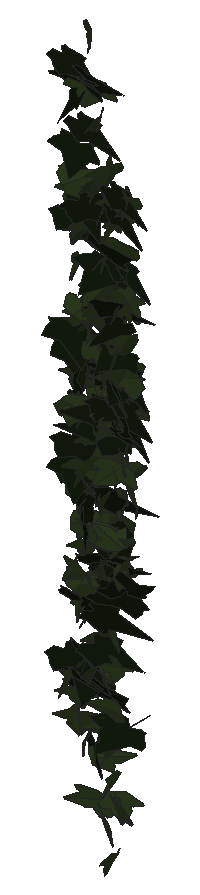
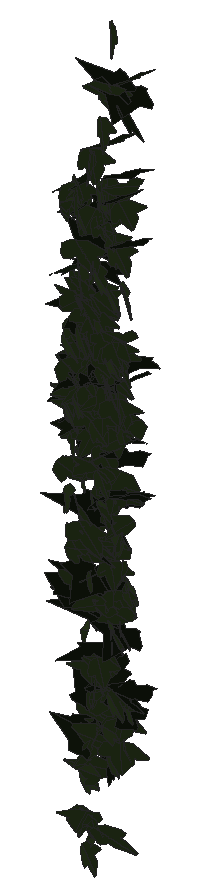
# SketchUp Ruby script. Lengths in millimetres.
U = 1.mm
M = Sketchup.active_model
def pt(a) = Geom::Point3d.new(a.map { |v| v * U })
def face(e, loops, mat)
  f = e.add_face(loops[0].map { |a| pt(a) })
  loops[1..].each { |l| e.add_face(l.map { |a| pt(a) }).erase! }
  f.material = f.back_material = mat if mat
  f
end
# faces: each face lists its corners as indices into pts; further lists are holes
def faces(e, pts, list, mat = nil) = list.each { |f| face(e, (f[0].is_a?(Array) ? f : [f]).map { |l| l.map { |i| pts[i] } }, mat) }
# xy, xz, yz: faces in a plane at the given z, y or x. An outline is a flat list of corners, or four numbers for a rectangle; further outlines are holes
def ring(l) = l.size == 4 ? [[l[0], l[1]], [l[2], l[1]], [l[2], l[3]], [l[0], l[3]]] : l.each_slice(2).to_a
def flat(e, list, mat, &to3) = list.each { |f| face(e, (f[0].is_a?(Array) ? f : [f]).map { |l| ring(l).map { |u, v| to3.(u, v) } }, mat) }
def xy(e, z, list, mat = nil) = flat(e, list, mat) { |x, y| [x, y, z] }
def xz(e, y, list, mat = nil) = flat(e, list, mat) { |x, z| [x, y, z] }
def yz(e, x, list, mat = nil) = flat(e, list, mat) { |y, z| [x, y, z] }
def lines(e, pts, list) = list.each { |a, b| e.add_line(pt(pts[a]), pt(pts[b])) }
# prism: a flat outline (further loops are holes) pulled along v
def prism(e, loops, v, mat = nil)
  f = face(e, loops, mat); d = Geom::Vector3d.new(v.map { |x| x * U })
  f.pushpull(f.normal.samedirection?(d) ? d.length : -d.length)
end
def box(e, o, s, mat = nil) = prism(e, [[o, [o[0] + s[0], o[1], o[2]], [o[0] + s[0], o[1] + s[1], o[2]], [o[0], o[1] + s[1], o[2]]]], [0, 0, s[2]], mat)
def at(x, y, z, deg = 0) = Geom::Transformation.translation(pt([x, y, z])) * Geom::Transformation.rotation(ORIGIN, Z_AXIS, deg.degrees)
def axes(o, x, y, z) = Geom::Transformation.new([*x, 0, *y, 0, *z, 0, *pt(o).to_a, 1])
def part(name) = M.definitions.add(name)
# library, detail: a bought-in or finely detailed component or shape, given as its bounding box
def library(name, o, s) = part(name).tap { |d| box(d.entities, o, s) }
def detail(e, o, s) = box(e.add_group.entities, o, s)
def put(e, d, t, mat = nil) = e.add_instance(d, t).tap { |i| i.material = mat if mat }
def group(e, t, mat = nil) = e.add_group.tap { |g| g.transformation = t; g.material = mat if mat }.entities
root = M.entities
M.materials.add("efeu1").color = [18, 25, 13]
M.materials.add("efeu2").color = [43, 57, 29]
c1 = part("ivyleaf_10")
p = [[0,12.8,-0.8],[-1.5,51.3,-10.9],[-4.9,51,-11.6],[-13.6,26.5,-7.3],[-13.2,15.9,-4.6],[-21.1,19.3,-7.2],
  [-29.5,16.3,-8.3],[-29.2,8.3,-6.2],[-19.7,-9.8,0.5],[-7.6,-13,4],[1,-12.2,5.8],[-0.4,51.1,-11.1],
  [-1.5,51.1,-10.9],[1,-12.4,5.9],[16.9,-12.4,3.5],[35.1,9.1,-5.1],[35,12.9,-6.1],[20.5,16.4,-4.9],
  [15.8,15,-3.8],[15.3,27.6,-7.1],[12.8,31.3,-7.8]]
faces(c1.entities,p,[[0,1,2,3,4,5,6,7,8,9,10],[11,12,0,13,14,15,16,17,18,19,20]],"efeu2")
c2 = part("ivyleaf_9")
p = [[39.1,54.8,31.7],[34.5,51.8,30.2],[-5.3,25.2,17.3],[-17.9,28.3,20.9],[-21.6,21.7,17],[-20.2,4.3,5.3],
  [-22.9,-0.3,2.5],[-17.1,-4,-0.6],[-2,-2.1,-1.2],[-0.7,-15.4,-10.1],[16.6,-22.3,-16.7],[21.1,-15.1,-12.5],
  [32.7,-10.7,-11],[46.1,-1.8,-6.6],[30.8,11.2,3.8]]
faces(c2.entities,p,[[0,1,2,3,4,5,6,7,8,9,10,11,12,13,14]],"efeu1")
put(root,c1,axes([1571.3,1015.9,668.1],[-0.2467,0.55616,-0.33098],[0.13791,-0.32296,-0.57106],[-1.22399,-0.14848,0.00237]))
put(root,c1,axes([1572.5,998.6,417.9],[0.27227,-0.40908,0.65552],[0.39143,-0.62245,-0.43333],[1.41754,0.25045,-0.00625]))
put(root,c1,axes([1567.8,1029,916.7],[-0.03546,-0.06959,0.70337],[0.65785,-0.61463,-0.05166],[1.17335,0.3425,0.05022]))
put(root,c1,axes([1580.5,1004,1147.2],[0.51099,-0.69659,-0.1656],[-0.05034,0.16709,-0.74574],[1.36176,0.26756,0.03457]))
put(root,c1,axes([1571.4,1008.6,747.9],[0.22223,0.32998,0.59583],[0.08777,0.5993,-0.34094],[-1.29329,0.09737,0.07924]))
put(root,c1,axes([1582.2,1024.8,1055.8],[-0.59959,-0.63157,0.16688],[0.03186,-0.19302,-0.69889],[1.24285,-0.29974,0.09842]))
put(root,c2,axes([1565.9,996.7,459.9],[0.02456,-0.40531,-0.66696],[0.0762,0.66651,-0.40426],[1.4834,-0.02753,0.03181]))
put(root,c1,axes([1588.2,1017.2,949.7],[-0.91985,-0.48124,0.19716],[-0.21237,-0.16693,-0.68099],[0.96674,-0.49457,0.03801]))
put(root,c1,axes([1590.5,1009.6,1027.6],[0.60365,-0.465,-0.45066],[-0.47859,0.37398,-0.56287],[1.1357,0.40476,0.00234]))
put(root,c1,axes([1596.5,991.9,612.7],[-0.91654,0.17381,0.41087],[-0.78506,0.05681,-0.50751],[-0.32341,-0.63048,0.06754]))
put(root,c2,axes([1565.1,1013.1,892.5],[0.76321,-0.45053,-0.46464],[-0.19004,0.49699,-0.56808],[1.21701,0.36015,0.20268]))
put(root,c1,axes([1583.8,1010.3,963.2],[0.10547,-0.61187,-0.33958],[0.00087,0.34067,-0.61377],[1.33183,0.04824,0.02729]))
put(root,c1,axes([1587.9,1017.7,1044.3],[-0.83524,-0.57309,0.04169],[-0.04203,-0.0356,-0.72181],[1.09278,-0.4394,0.00411]))
put(root,c1,axes([1587.8,1005.5,349],[-1.17604,-0.44909,0.02119],[-0.02351,-0.01904,-0.76384],[0.85533,-0.618,0.00814]))
put(root,c1,axes([1575.5,989.2,606.3],[0.26339,-0.66648,-0.11301],[0.11433,-0.10277,0.67967],[-1.28146,-0.14616,0.03741]))
put(root,c1,axes([1587,999.9,1288.4],[-0.53752,-0.66214,0.27353],[0.05023,-0.30344,-0.70728],[1.36255,-0.25002,0.13398]))
put(root,c1,axes([1589.3,1009.9,1217.6],[-0.27287,-0.74091,0.11093],[-0.08269,-0.10453,-0.75431],[1.42341,-0.14811,-0.02255]))
put(root,c2,axes([1568.6,1000.1,1235.9],[0.23567,-0.64879,-0.39765],[0.10163,0.4093,-0.65116],[1.44469,0.07704,0.11068]))
put(root,c2,axes([1576.8,1001.7,1031.5],[-0.70551,-0.6188,-0.35039],[0.3314,0.30413,-0.72131],[1.31219,-0.40951,-0.00623]))
put(root,c2,axes([1581.7,1007.6,1354.6],[-0.62223,-0.68562,0.137],[-0.02858,-0.14432,-0.75808],[1.33037,-0.32377,0.04779]))
put(root,c1,axes([1586.6,1000.9,394.3],[-1.05283,-0.3505,-0.07329],[0.1308,0.02845,-0.65476],[0.66884,-0.5573,0.01268]))
put(root,c1,axes([1587.9,1023.6,442.5],[0.18433,-0.70342,0.15714],[0.01915,-0.15722,-0.70997],[1.37161,0.09673,-0.01121]))
put(root,c2,axes([1574.7,1001.1,995.3],[-0.08397,-0.79522,-0.04255],[0.01864,0.04207,-0.79641],[1.51552,-0.04458,0.00744]))
put(root,c1,axes([1583.5,1021.2,717.2],[-0.12826,-0.12145,-0.66567],[-0.04806,-0.66804,0.12444],[-1.28692,0.03705,0.06169]))
put(root,c2,axes([1582.3,1002.9,789.2],[-0.56018,-0.71563,-0.02349],[0.00585,0.02413,-0.77377],[1.36271,-0.29428,-0.00633]))
put(root,c1,axes([1586.4,1023.7,560.4],[0.78746,-0.60576,0.09546],[0.07673,-0.08804,-0.7334],[1.16459,0.4154,-0.01623]))
put(root,c2,axes([1593.9,994.6,1457],[-0.93924,0.41452,-0.46805],[0.70275,-0.28796,-0.64435],[-0.96024,-0.6162,-0.01375]))
put(root,c2,axes([1581.6,1003.3,557.9],[1.39909,0.05142,-0.30835],[-0.586,-0.0172,-0.73691],[-0.10292,0.79699,0.00399]))
put(root,c1,axes([1608,1020.9,201.7],[0.70546,-0.02856,-0.60696],[-1.14695,0.07369,-0.3715],[0.14797,0.70737,0.0142]))
put(root,c1,axes([1591.6,1026,1038.5],[0.17746,-0.70303,0.1308],[-0.00469,-0.13222,-0.70892],[1.36096,0.09122,-0.0195]))
put(root,c2,axes([1569.1,986.4,1518.5],[0.61992,-0.67329,-0.30174],[0.10223,0.3506,-0.72433],[1.40047,0.27244,0.18644]))
put(root,c1,axes([1614.5,1006,995.7],[-0.65115,0.0281,0.67312],[-1.27638,0.05762,-0.34329],[-0.122,-0.75288,-0.00115]))
put(root,c1,axes([1573.3,1008.9,352.7],[0.49889,-0.2531,0.68432],[0.89549,-0.4971,-0.36409],[1.0613,0.53842,-0.01447]))
put(root,c1,axes([1580.2,1009.3,555.1],[0.65025,-0.49758,0.39293],[0.52117,-0.28676,-0.60125],[1.08831,0.43462,0.05315]))
put(root,c1,axes([1588.3,1003.6,706.9],[-0.61576,0.56651,-0.06615],[0.05381,-0.06003,-0.65237],[-1.08418,-0.32473,0.00519]))
put(root,c1,axes([1580.6,1005.9,1062.6],[0.63518,0.32461,-0.59421],[0.64135,0.49497,0.45966],[1.11772,-0.46848,0.07392]))
put(root,c2,axes([1592.5,980.9,1489.2],[1.27558,0.40751,-0.24645],[-0.58004,0.04008,-0.76257],[-0.69647,0.71298,0.18372]))
put(root,c1,axes([1595.2,1003.9,799.4],[-0.8837,-0.61169,-0.19589],[0.22243,0.15722,-0.76796],[1.202,-0.4788,-0.00191]))
put(root,c2,axes([1576.2,1003.4,793.3],[0.05356,-0.46715,-0.61659],[0.38556,0.59991,-0.44527],[1.42088,-0.14518,0.14407]))
put(root,c1,axes([1617.8,1006.7,790.2],[0.31984,0.13555,-0.7043],[-1.33673,-0.11542,-0.1898],[-0.27648,0.71482,0.10291]))
put(root,c1,axes([1597.6,1020,384.8],[0.0955,-0.44885,0.47814],[0.05266,-0.47767,-0.4513],[1.24703,0.05454,-0.01756]))
put(root,c2,axes([1565.9,1002.4,409.2],[0.66335,-0.25759,0.64088],[0.94752,-0.40389,-0.43309],[0.91119,0.60752,-0.0162]))
put(root,c1,axes([1601.8,999.5,767.3],[-0.70343,0.47797,0.25833],[-0.3528,0.18275,-0.60335],[-0.97199,-0.41224,0.03205]))
put(root,c1,axes([1602.2,1002.3,1224.4],[-0.12873,-0.69563,0.2869],[-0.05495,-0.28544,-0.69891],[1.43105,-0.07353,-0.00103]))
put(root,c1,axes([1594.3,1002.6,820.7],[-1.11835,-0.30404,-0.24429],[0.4034,0.12187,-0.66153],[0.62311,-0.62459,-0.01016]))
put(root,c1,axes([1601.8,992.3,1221.6],[-0.04665,-0.64527,-0.38576],[0.03603,0.38531,-0.64572],[1.43034,-0.03075,0.00369]))
put(root,c1,axes([1593.6,1020.9,1060.4],[-1.30245,0.04444,-0.22898],[0.42736,-0.06655,-0.68402],[-0.12013,-0.71856,0.04919]))
put(root,c1,axes([1603.3,1006.2,659.3],[-0.68482,-0.54915,-0.00647],[0.00771,0.00508,-0.65654],[1.0452,-0.35985,0.0006]))
put(root,c1,axes([1619.9,1013.9,423.1],[-0.0077,0.02322,0.68184],[-0.9832,-0.44547,0.01211],[0.84809,-0.51622,0.02022]))
put(root,c2,axes([1584.8,1000.5,1311.1],[0.2239,-0.7227,-0.23839],[0.07044,0.24637,-0.72862],[1.44662,0.09986,0.07237]))
put(root,c1,axes([1582.7,982,909.9],[-0.65632,-0.23576,-0.59298],[1.07831,0.19698,-0.40782],[0.55875,-0.65707,0.0905]))
put(root,c2,axes([1622.8,985.3,740.5],[-0.2949,0.04401,-0.79776],[-1.42065,0.28179,0.16053],[0.54221,0.76225,-0.01329]))
put(root,c1,axes([1605,989.6,900.5],[0.24019,-0.5809,-0.46086],[-0.02731,0.46549,-0.59066],[1.41098,0.1079,0.06702]))
put(root,c2,axes([1602.7,982.1,945.8],[-0.09331,-0.34116,0.7374],[0.63201,0.66581,0.33012],[-1.41128,0.32072,0.09908]))
put(root,c1,axes([1593.2,1009.1,887.5],[-0.86768,0.42668,-0.33487],[0.49644,-0.21107,-0.62406],[-0.90507,-0.52482,-0.02127]))
put(root,c1,axes([1606,997.7,796.2],[0.14635,-0.63436,0.29675],[0.02975,-0.29691,-0.63874],[1.33256,0.0763,-0.01833]))
put(root,c1,axes([1603.1,1011.6,975.8],[0.46632,-0.65295,0.10297],[0.12903,-0.08441,-0.69661],[1.25142,0.25202,0.03346]))
put(root,c1,axes([1585.2,1004.6,577.6],[0.85818,0.17818,-0.53629],[0.92631,0.22619,0.48438],[0.54654,-0.66315,0.02112]))
put(root,c1,axes([1591.3,969.3,1310.3],[0.40457,0.04788,-0.83473],[0.79836,0.73893,0.14921],[1.3765,-0.44265,0.15879]))
put(root,c1,axes([1598.2,1004,307],[0.13502,-0.52051,-0.47781],[0.118,-0.47378,0.52532],[-1.33955,-0.0942,-0.00189]))
put(root,c1,axes([1605.3,1014.2,939.5],[-1.23924,-0.28772,0.04328],[0.0754,0.01742,0.71187],[-0.54858,0.65234,0.00007]))
put(root,c2,axes([1591.3,983.4,851.5],[0.01509,-0.53012,-0.6409],[0.11299,0.63966,-0.52835],[1.57892,-0.04071,0.04393]))
put(root,c1,axes([1609.6,995.4,542],[0.06522,-0.53437,-0.42188],[-0.04824,0.42112,-0.53546],[1.29486,0.0426,0.0013]))
put(root,c1,axes([1609.7,1023.8,825.1],[-0.13731,-0.67541,0.00443],[-0.00083,-0.00441,-0.67925],[1.28547,-0.07215,0.00003]))
put(root,c1,axes([1624.2,1011.9,692.5],[0.39541,0.02341,0.63738],[-1.07162,0.32162,0.17172],[-0.57021,-0.5882,0.11926]))
put(root,c1,axes([1604.9,1020.7,752],[0.842,-0.57961,0.13419],[0.17495,-0.09863,-0.72905],[1.1187,0.45167,0.01301]))
put(root,c1,axes([1632.5,1000.6,1010.6],[-0.15151,0.11088,-0.75229],[-1.13544,0.4599,0.13092],[0.89735,0.60064,0.03863]))
put(root,c2,axes([1609,1006,436.4],[-1.27421,-0.24336,-0.3516],[0.63678,0.10861,-0.71228],[0.50676,-0.74838,0.01096]))
put(root,c1,axes([1609,1008.2,754.3],[0.38905,-0.52267,0.41884],[-0.21991,0.40382,0.56033],[-1.25562,-0.23267,0.03164]))
put(root,c1,axes([1614.1,1021.9,493.3],[-0.44914,-0.6555,-0.03047],[0.01887,0.02881,-0.69668],[1.24875,-0.2362,-0.00043]))
put(root,c1,axes([1610.6,999.3,1130],[0.40498,-0.68285,0.183],[0.11994,-0.17203,-0.71519],[1.34011,0.22176,0.0087]))
put(root,c1,axes([1592.5,981.3,886.6],[0.31166,0.18074,-0.77114],[1.04295,0.5427,0.24357],[1.08837,-0.5718,-0.01258]))
put(root,c2,axes([1595.2,990.1,477.4],[1.19235,-0.45291,-0.16641],[-0.23326,0.11441,-0.77279],[0.88821,0.63804,0.02045]))
put(root,c1,axes([1617.1,1005.4,979.9],[0.43032,-0.62599,-0.27759],[-0.12665,0.27086,-0.66502],[1.29711,0.23412,0.02716]))
put(root,c2,axes([1601.2,995,1264.4],[0.07248,-0.75422,-0.13087],[0.0016,0.13107,-0.75514],[1.45688,0.03738,0.00734]))
put(root,c2,axes([1600.3,999.4,706.6],[0.00336,0.03083,-0.81568],[1.22518,-0.50157,-0.01757],[-0.95516,-0.64325,-0.0254]))
put(root,c2,axes([1594.2,995.3,1404.3],[0.66412,-0.64737,-0.28217],[0.14647,0.34773,-0.70259],[1.33602,0.28368,0.21729]))
put(root,c1,axes([1622.1,1002.5,854.5],[-0.42511,-0.71318,0.13099],[-0.05855,-0.12762,-0.74729],[1.37879,-0.22531,0.00865]))
put(root,c1,axes([1615.8,992.3,1481.4],[1.50711,0.13106,-0.06373],[-0.16595,0.14394,-0.7874],[-0.22223,0.78129,0.15576]))
put(root,c1,axes([1601.6,1020.6,603.3],[-0.5033,0.16571,0.61709],[1.0073,-0.31735,0.31203],[0.68128,0.59163,-0.00547]))
put(root,c1,axes([1622,997,448.7],[-0.00335,-0.69906,-0.01878],[-0.00164,0.01878,-0.69906],[1.33093,-0.00174,-0.00091]))
put(root,c1,axes([1610.4,989.1,595.5],[-0.25306,-0.31212,-0.56424],[0.62069,0.46444,-0.33377],[1.05868,-0.3469,0.06081]))
put(root,c1,axes([1622.2,1021.5,904.7],[-0.08943,-0.63792,0.26533],[0.0396,-0.26713,-0.63856],[1.31432,-0.03536,0.03729]))
put(root,c1,axes([1625.6,1003.9,1252.3],[-0.35882,-0.70896,0.17471],[-0.05715,-0.17276,-0.73345],[1.38849,-0.19032,0.01496]))
put(root,c1,axes([1623.5,988.4,1314.1],[-0.07854,-0.73984,-0.2799],[0.04395,0.27904,-0.74096],[1.50483,-0.04676,0.00703]))
put(root,c1,axes([1626.5,1007.6,1116.7],[-0.34927,-0.59789,0.55946],[-0.00207,-0.57316,-0.61289],[1.55838,-0.13476,0.12457]))
put(root,c1,axes([1625.5,1000.8,1421.5],[0.01946,-0.72779,-0.29579],[0.02119,0.29592,-0.72772],[1.495,0.00528,0.01417]))
put(root,c1,axes([1627.1,1005.5,1088.3],[-0.05512,-0.72983,0.18529],[-0.05646,-0.18417,-0.73008],[1.43196,-0.03535,-0.02165]))
put(root,c1,axes([1622.5,980.2,1580.1],[0.62489,-0.67979,-0.3174],[0.11922,0.37009,-0.72785],[1.42287,0.26754,0.20038]))
put(root,c1,axes([1613.8,1000.8,474.8],[-0.2191,-0.43546,0.48275],[0.35948,0.44671,0.448],[-1.18397,0.21622,0.04669]))
put(root,c1,axes([1625.2,1011.2,1162.9],[0.3163,-0.70962,0.2174],[0.07789,-0.21368,-0.72877],[1.41035,0.17094,-0.00851]))
put(root,c1,axes([1594.7,999.3,693.1],[0.09216,-0.13103,-0.80215],[1.54676,0.01812,0.0461],[0.01985,-0.80341,0.13187]))
put(root,c1,axes([1620.4,999,942.4],[0.00768,0.08553,0.81445],[-0.00587,0.81446,-0.08551],[-1.55858,-0.00265,0.00434]))
put(root,c2,axes([1594.3,989.5,1487.1],[1.06579,-0.05485,-0.58043],[1.09991,0.15828,0.54263],[0.14621,-0.79085,0.14886]))
put(root,c1,axes([1626.6,1000.6,1299.2],[0.27605,-0.72586,0.23756],[0.14443,-0.22691,-0.73966],[1.44637,0.16119,0.02852]))
put(root,c2,axes([1644.8,997.1,903.1],[-0.53479,-0.19036,0.68548],[-1.12185,-0.35034,-0.33893],[0.75807,-0.65276,-0.018]))
put(root,c2,axes([1609.2,1002.2,314.1],[-0.05346,-0.00164,-0.77935],[1.36707,-0.30263,-0.02525],[-0.57548,-0.71874,0.01241]))
put(root,c1,axes([1636.4,1014.2,913.9],[-1.05965,-0.39305,0.14413],[-0.21844,-0.08733,-0.68151],[0.76623,-0.56846,0.00504]))
put(root,c1,axes([1647.3,1003.9,1082.9],[-1.12615,-0.00433,0.43275],[-0.81845,-0.07642,-0.58877],[0.09248,-0.72908,0.05914]))
put(root,c2,axes([1622.2,1036.6,649.2],[-0.3212,-0.72254,0.32211],[-0.05478,-0.32353,-0.74081],[1.50459,-0.16602,0.04179]))
put(root,c1,axes([1628,1016.5,1082.7],[-0.4674,-0.68107,-0.07656],[0.3033,0.02235,-0.71002],[1.26862,-0.25627,0.14154]))
put(root,c1,axes([1634.5,994.6,1271.3],[0.47976,-0.59286,-0.41994],[-0.16341,0.41707,-0.64035],[1.37302,0.2568,0.07052]))
put(root,c1,axes([1648.1,1007.7,675.7],[0.78134,0.32726,0.60215],[-0.95486,-0.33465,0.52395],[0.88854,-0.64741,0.03355]))
put(root,c2,axes([1612.7,975.6,1279.3],[0.14465,-0.21616,-0.78369],[0.24959,0.78005,-0.20244],[1.52694,-0.10703,0.10733]))
put(root,c1,axes([1650.2,1020,716.6],[-1.16243,-0.01599,0.45563],[-0.86607,-0.02519,-0.61089],[0.05306,-0.76159,0.01064]))
put(root,c1,axes([1639.2,990.4,1298.5],[0.36636,-0.14738,-0.75254],[-0.26282,0.75655,-0.18349],[1.43559,0.17612,0.15845]))
put(root,c1,axes([1635.1,1011.3,632.2],[-0.00377,-0.71401,0.02879],[-0.00053,-0.02879,-0.71401],[1.36001,-0.00199,-0.0002]))
put(root,c1,axes([1637.6,1012.9,1089.3],[-1.30772,-0.24609,0.07687],[-0.05058,-0.15006,-0.71789],[0.48806,-0.67492,0.13158]))
put(root,c1,axes([1634.2,1012.7,411.1],[-1.04545,0.49453,0.16703],[0.22685,-0.11723,0.73909],[0.96717,0.56205,0.0072]))
put(root,c1,axes([1639.2,1016.9,958.4],[-0.58551,-0.53858,0.33019],[-0.03999,-0.35834,-0.60406],[1.20166,-0.27435,0.14079]))
put(root,c1,axes([1611.8,1019.2,597.2],[0.80192,0.17662,0.56812],[0.99933,0.21693,-0.45687],[-0.53239,0.67323,-0.00183]))
put(root,c1,axes([1629.6,991.3,828.7],[-0.34699,-0.42263,-0.67037],[0.58027,0.59753,-0.45963],[1.39214,-0.3544,0.02449]))
put(root,c1,axes([1645.5,994.2,435.7],[-0.36787,0.29154,0.5715],[-0.61019,0.47311,-0.34978],[-1.05763,-0.37436,0.00302]))
put(root,c1,axes([1636.6,1008.2,1178.5],[0.27791,-0.66038,-0.36155],[0.19075,0.38206,-0.65736],[1.42011,0.07792,0.15905]))
put(root,c2,axes([1665.3,996.7,874.4],[-0.49502,-0.35452,-0.67933],[-0.76045,-0.5494,0.4397],[-1.24441,0.47676,0.00154]))
put(root,c1,axes([1663.2,1007.5,348],[-0.29072,-0.12758,0.73648],[-1.09781,-0.45793,-0.19896],[0.90467,-0.59669,-0.00477]))
put(root,c1,axes([1635.7,1010,881.4],[-0.53829,-0.59362,-0.3974],[0.46928,0.32002,-0.65353],[1.27602,-0.36812,0.0727]))
put(root,c2,axes([1635,1007.5,636.5],[0.83921,0.61111,0.25887],[0.28355,0.21171,-0.75358],[-1.23087,0.46543,0.0029]))
put(root,c1,axes([1638.4,1005,284.4],[0.22775,-0.41084,0.50869],[-0.12769,0.50669,0.42501],[-1.23788,-0.12786,0.04975]))
put(root,c1,axes([1665.6,992.3,389.6],[-0.29408,0.03496,0.65248],[-1.24341,0.00265,-0.15486],[-0.02024,-0.67052,0.03341]))
put(root,c2,axes([1651.9,994.7,1167.4],[-1.3266,-0.32432,-0.00813],[0.01209,0.00563,-0.76879],[0.61732,-0.69706,-0.00243]))
put(root,c1,axes([1641.9,1007.1,1262.3],[-1.42187,0.08307,-0.09765],[0.18103,-0.02795,-0.7515],[-0.16359,-0.75293,0.01712]))
put(root,c1,axes([1640.1,990.7,1097.2],[-0.6875,-0.53791,-0.39888],[0.38279,0.34514,-0.64759],[1.21566,-0.41289,-0.02167]))
put(root,c1,axes([1645.3,995.1,762.5],[0.16811,-0.66073,-0.05134],[0.0024,0.05197,-0.66655],[1.26128,0.08797,0.00811]))
put(root,c1,axes([1643.4,1023.7,1110.7],[1.03473,-0.49134,-0.04819],[-0.04928,0.04321,-0.73266],[0.93831,0.5441,0.01466]))
put(root,c2,axes([1613.3,1008.2,620.9],[0.43145,-0.16259,0.72341],[1.36834,-0.13668,-0.25602],[0.34488,0.74567,0.11081]))
put(root,c1,axes([1640.1,995.9,357],[-0.04343,0.31728,-0.58082],[0.0006,-0.58116,-0.31748],[-1.2596,-0.01121,0.01987]))
put(root,c1,axes([1623.7,1022.8,827.3],[0.97023,0.06693,0.47907],[0.91056,0.03285,-0.5137],[-0.13574,0.69879,-0.02174]))
put(root,c2,axes([1674.6,1004.6,690],[-0.64463,0.01213,-0.73003],[-1.38772,0.03596,0.3389],[0.07179,0.80397,-0.00415]))
put(root,c1,axes([1651.1,1010.1,924.8],[1.24937,-0.03582,-0.25665],[-0.48252,0.05584,-0.65627],[0.10204,0.70263,0.03907]))
put(root,c1,axes([1661.2,1011.7,1200.4],[-1.22977,-0.24459,0.32201],[-0.53636,-0.16292,-0.68926],[0.55191,-0.70333,0.04768]))
put(root,c1,axes([1646.1,1003.3,1122.6],[0.15432,-0.47044,-0.55535],[0.20198,0.56046,-0.45928],[1.3704,-0.02963,0.13023]))
put(root,c1,axes([1645.8,1001,1355.6],[0.39515,-0.65917,-0.37428],[0.19367,0.40879,-0.6635],[1.42959,0.12682,0.19334]))
put(root,c1,axes([1627.7,992.2,1020.5],[1.06675,-0.2042,0.53557],[0.94301,-0.20395,-0.59632],[0.54839,0.74793,-0.01638]))
put(root,c1,axes([1642.1,997.7,181.4],[-0.43286,0.52827,-0.27261],[0.20622,-0.25015,-0.57515],[-1.11242,-0.25193,-0.00054]))
put(root,c2,axes([1664.1,990.6,888.6],[0.43127,-0.22521,0.70442],[-0.73235,0.59326,0.31346],[-1.20198,-0.44227,0.06176]))
put(root,c1,axes([1649.8,999.3,894.8],[0.13451,-0.50987,0.49944],[0.17508,-0.49119,-0.51447],[1.34704,0.11476,0.01699]))
put(root,c1,axes([1652.7,1008.4,1048.9],[0.85917,-0.5573,-0.11008],[-0.10022,0.09895,-0.71689],[1.07649,0.45401,0.02112]))
put(root,c1,axes([1644.7,1001.2,468.9],[1.15491,0.27232,0.03624],[0.06226,0.01563,-0.66513],[-0.51913,0.6077,0.00087]))
put(root,c1,axes([1669.5,987.5,472.4],[0.48738,-0.21754,-0.58474],[-0.85233,0.37598,-0.33601],[0.8267,0.51588,-0.00169]))
put(root,c1,axes([1656.4,1008.1,212.5],[-1.02361,0.44317,0.1226],[-0.18889,0.07233,-0.69686],[-0.85448,-0.54687,0.00718]))
put(root,c1,axes([1667.5,1011.7,1132.9],[0.87912,-0.34658,-0.50755],[-0.78986,0.2924,-0.57737],[0.86274,0.62087,-0.01141]))
put(root,c2,axes([1676.5,1003.4,593.7],[0.23333,0.11441,-0.79143],[-1.21173,-0.47048,-0.16664],[-0.92083,0.6481,0.01875]))
put(root,c1,axes([1631.4,996.4,295.1],[0.27471,0.05661,-0.72448],[1.17763,0.37775,0.15279],[0.72524,-0.63483,0.02632]))
put(root,c2,axes([1650.8,990.7,884.7],[1.26881,0.21685,-0.31888],[-0.57495,-0.10214,-0.70104],[-0.45615,0.73192,-0.00335]))
put(root,c1,axes([1657.1,1014.4,1051.4],[0.08126,-0.71689,-0.05118],[-0.01997,0.05065,-0.71812],[1.36772,0.04333,-0.00744]))
put(root,c2,axes([1633.8,986.7,497.2],[0.29111,-0.26991,-0.70732],[0.33708,0.71435,-0.23429],[1.40087,-0.1158,0.20336]))
put(root,c1,axes([1659.8,1001.2,799.3],[0.02517,0.0485,-0.70903],[-0.13951,0.70546,0.04689],[1.34537,0.07225,0.01813]))
put(root,c1,axes([1650.6,998.9,324.3],[-0.08495,-0.34452,-0.63146],[0.3662,0.6039,-0.34309],[1.31914,-0.18983,0.05458]))
put(root,c1,axes([1629.5,1018.8,203.2],[0.44829,-0.03678,0.64673],[1.22012,-0.08536,-0.23835],[0.17665,0.68297,0.00504]))
put(root,c2,axes([1665.3,996.8,993.7],[0.55187,0.457,-0.549],[-0.53908,-0.47037,-0.54116],[-1.24804,0.40525,-0.00901]))
put(root,c1,axes([1663.2,998.3,900],[-0.70794,-0.52217,0.42701],[-0.20019,-0.43677,-0.62573],[1.26807,-0.36047,0.13961]))
put(root,c1,axes([1659.1,985.9,1348.3],[-0.54398,-0.74303,-0.05137],[0.01696,0.0516,-0.79604],[1.4174,-0.28578,-0.01019]))
put(root,c1,axes([1652.6,1029.4,942.4],[0.27311,-0.62167,0.28578],[0.24794,-0.26183,-0.63499],[1.27837,0.18359,0.0621]))
put(root,c2,axes([1625.5,1005.8,751.1],[0.65324,0.18713,-0.67012],[1.03811,0.3915,0.38871],[0.82204,-0.64311,0.04164]))
put(root,c1,axes([1648.2,1017.1,218.1],[0.93155,0.51408,0.11966],[0.1572,0.08658,-0.70982],[-0.99217,0.49639,-0.00011]))
put(root,c1,axes([1667.2,994.2,686.2],[0.42358,0.55719,0.38691],[-0.38946,-0.33308,0.59738],[1.23088,-0.29713,0.05587]))
put(root,c1,axes([1646.9,1005.4,666.8],[-1.19207,-0.02502,0.39526],[0.75375,-0.04365,0.62483],[0.00416,0.73935,0.05026]))
put(root,c1,axes([1653.8,992.1,990.3],[-0.12997,-0.37127,-0.64158],[0.44588,0.60046,-0.37242],[1.33845,-0.23608,0.06176]))
put(root,c1,axes([1667.2,995.2,816.5],[1.31304,0.05647,-0.35141],[-0.66421,-0.04314,-0.6921],[-0.13298,0.77305,-0.01295]))
put(root,c1,axes([1662.2,1000.1,1250.3],[0.1322,-0.67362,0.33681],[0.03882,-0.33643,-0.67707],[1.43283,0.07127,-0.01273]))
put(root,c1,axes([1654.8,997.5,949.4],[0.00802,0.30158,0.77044],[0.07223,0.76956,-0.30145],[-1.57297,0.03687,-0.00991]))
put(root,c1,axes([1666.7,989.8,907.1],[-1.23369,0.50048,0.01064],[0.0151,-0.00713,0.81894],[0.95261,0.64827,0.00079]))
put(root,c2,axes([1643,998.6,409.3],[-0.2973,-0.22394,0.73655],[0.77418,-0.66208,-0.11503],[1.24392,0.35854,0.24763]))
put(root,c2,axes([1641.7,1013.1,970.5],[-0.38782,-0.328,-0.71954],[0.99487,0.50167,-0.37672],[1.12927,-0.55461,0.08478]))
put(root,c1,axes([1653.2,1021.5,754],[0.87614,-0.45205,0.31976],[0.46449,-0.2076,-0.64487],[0.94592,0.52064,0.02049]))
put(root,c2,axes([1661.8,992.4,971],[0.79168,-0.24378,-0.60507],[-0.93529,0.35481,-0.4808],[0.81645,0.64284,0.03592]))
put(root,c1,axes([1666.4,988.6,135],[0.05991,-0.74668,0.07871],[0.01569,-0.07843,-0.74732],[1.42886,0.03217,0.00491]))
put(root,c2,axes([1641.1,995.5,1190.5],[-0.14287,-0.22955,0.73009],[0.92697,-0.58019,-0.13234],[1.12353,0.44949,0.20203]))
put(root,c1,axes([1663.8,995.3,270.4],[0.23394,-0.58224,0.4466],[0.15983,-0.43869,-0.59504],[1.38739,0.14871,-0.00676]))
put(root,c1,axes([1668.7,1000,1153.6],[0.14169,-0.66199,-0.38008],[-0.0333,0.3803,-0.6658],[1.45241,0.0733,0.02181]))
put(root,c1,axes([1674.1,983.8,515.6],[-0.12207,0.37584,-0.55475],[-0.27323,0.53663,0.38017],[1.24567,0.15454,0.02902]))
put(root,c1,axes([1663.9,997.4,936.5],[-0.83612,0.63393,0.00103],[-0.00121,0.00081,-0.77128],[-1.2065,-0.43932,0.00006]))
put(root,c2,axes([1639.8,980.6,1099.9],[1.19551,0.17577,0.47658],[0.88606,0.1039,-0.65196],[-0.38663,0.78161,-0.02051]))
put(root,c2,axes([1660.6,1008.4,960.8],[-0.35575,-0.53612,0.58713],[-0.11435,-0.59189,-0.5596],[1.50887,-0.17126,0.09602]))
put(root,c2,axes([1672.4,1000.8,1070.7],[-0.09984,-0.06216,-0.76835],[0.40489,-0.74139,0.04546],[-1.41012,-0.20847,0.06745]))
put(root,c1,axes([1669.7,1002.1,1270.9],[0.04642,-0.72301,-0.23447],[0.08832,0.23557,-0.72157],[1.44388,0.00883,0.05168]))
put(root,c1,axes([1668.8,1003.7,1107],[0.42366,-0.68689,0.17507],[0.07757,-0.17079,-0.72193],[1.34685,0.2259,-0.01349]))
put(root,c2,axes([1655.3,1006.9,335.1],[0.26943,0.74264,0.09302],[-0.06795,-0.08786,0.75579],[1.42281,-0.14482,0.01848]))
put(root,c2,axes([1638,981.5,558.5],[0.45239,-0.03307,-0.74369],[1.1316,0.47819,0.16877],[0.85251,-0.61718,0.17062]))
put(root,c1,axes([1656,991.9,885.2],[-0.87376,-0.31267,-0.53001],[0.88211,0.25928,-0.55443],[0.77038,-0.6515,0.03372]))
put(root,c1,axes([1668.5,1014.2,618.6],[-0.45636,-0.59809,-0.16156],[-0.11277,-0.1503,0.64437],[-1.17368,0.247,0.00091]))
put(root,c1,axes([1670.8,1019.2,674.6],[0.05577,-0.2607,0.61197],[0.06167,-0.61128,-0.26196],[1.26448,0.04131,-0.01421]))
put(root,c1,axes([1693.4,992.3,987.5],[0.83423,-0.10027,-0.70539],[-1.27996,0.2152,-0.4485],[0.44768,0.80212,0.03215]))
put(root,c2,axes([1676.1,1000.1,1025.7],[-0.84218,-0.50001,0.42613],[-0.32044,-0.41031,-0.65629],[1.20857,-0.45722,0.12294]))
put(root,c1,axes([1678,1020.1,991],[-0.54831,-0.54663,0.41472],[-0.12943,-0.42483,-0.6072],[1.29944,-0.27297,0.11451]))
put(root,c1,axes([1676.1,1000.7,1290],[-0.90086,-0.61308,0.07744],[0.00691,-0.1003,-0.77191],[1.17607,-0.46903,0.06385]))
put(root,c1,axes([1670.3,996,630.7],[-0.07032,0.6081,0.31425],[-0.1108,0.31078,-0.60823],[-1.29803,-0.05947,0.03489]))
put(root,c1,axes([1674.3,1022.8,917.2],[0.37698,-0.684,0.06765],[0.00823,-0.06916,-0.71194],[1.30811,0.19756,-0.01502]))
put(root,c1,axes([1675.1,978.6,1034.5],[0.41049,-0.58287,-0.42597],[0.02567,0.44775,-0.60584],[1.37375,0.1658,0.1386]))
put(root,c1,axes([1676.8,1012.2,980.2],[0.50501,-0.66463,-0.08562],[-0.04413,0.08293,-0.71558],[1.27462,0.2662,0.00915]))
put(root,c1,axes([1666.2,1017.4,918.6],[1.37029,-0.04013,0.1171],[0.22252,-0.0064,-0.72111],[0.07734,0.72943,0.00012]))
put(root,c2,axes([1686.2,995.8,364.8],[-1.32528,-0.38468,0.06883],[-0.10259,-0.04474,-0.79543],[0.73664,-0.69831,0.01305]))
put(root,c1,axes([1649,1013.1,941.7],[0.52825,0.03968,0.66509],[1.22559,0.16892,-0.27882],[-0.32541,0.70061,0.02956]))
put(root,c2,axes([1672.9,1004.2,594.1],[1.07276,0.27199,0.51151],[-0.91094,-0.18343,0.62498],[0.62117,-0.73872,0.03315]))
put(root,c1,axes([1680.3,989.7,997.8],[-0.5019,-0.699,-0.02829],[0.00825,0.0286,-0.74707],[1.33141,-0.26368,-0.00604]))
put(root,c1,axes([1687.2,996.7,854.3],[-0.23329,0.50345,0.43],[-0.6168,0.33572,-0.48545],[-1.09882,-0.29534,0.1812]))
put(root,c1,axes([1686.7,1020.3,814.3],[-0.28754,-0.48311,0.45298],[-0.22257,-0.43786,-0.50598],[1.24061,-0.19053,0.01421]))
put(root,c2,axes([1661.3,1007.9,1170.4],[0.5522,-0.67865,-0.19584],[0.02812,0.21751,-0.73183],[1.34402,0.27428,0.09577]))
put(root,c2,axes([1662.3,996.5,1273.1],[0.61834,-0.69303,-0.09297],[-0.06067,0.08773,-0.76537],[1.32941,0.32635,0.00831]))
put(root,c1,axes([1684.5,997.1,1051.4],[-0.42565,-0.67746,0.1323],[-0.04732,-0.13107,-0.71321],[1.31284,-0.22437,0.01719]))
put(root,c1,axes([1660.1,1015.7,1110.1],[1.13685,-0.02776,0.42573],[0.81196,0.03741,-0.59616],[0.00162,0.73257,0.04658]))
put(root,c1,axes([1665,1005.8,834],[0.15039,-0.18303,0.63821],[0.85436,-0.45882,-0.18716],[0.93101,0.45061,0.06866]))
put(root,c1,axes([1683.5,1013.1,1032],[0.09106,-0.6977,0.13138],[-0.02376,-0.13249,-0.69902],[1.351,0.04469,-0.02115]))
put(root,c1,axes([1650.5,1007,933.8],[-0.02787,-0.08882,0.80825],[1.54672,-0.02753,0.0117],[0.04965,0.80791,0.08925]))
put(root,c1,axes([1681.6,994.3,1294.6],[0.63761,-0.66947,-0.18556],[0.01701,0.21014,-0.74204],[1.32207,0.32017,0.09904]))
put(root,c1,axes([1691.3,1009.9,1268],[-0.45225,0.60828,-0.39892],[-0.28797,0.36915,0.65302],[1.35415,0.28165,0.00565]))
put(root,c1,axes([1693.1,1009.9,1266.7],[-0.33535,0.49277,-0.55862],[-0.39415,0.519,0.52314],[1.3618,0.27156,0.01385]))
put(root,c2,axes([1657.4,988.6,932.9],[-0.1739,-0.30954,-0.73597],[1.05638,0.50785,-0.28251],[1.09227,-0.54045,0.15606]))
put(root,c1,axes([1690.2,1007.8,757.9],[0.30124,-0.04817,-0.76931],[-0.29683,0.76712,-0.08012],[1.43667,0.16859,0.14476]))
put(root,c2,axes([1664.3,989.8,1310],[0.69054,-0.64485,-0.2374],[-0.03874,0.25826,-0.73262],[1.30723,0.34829,0.10369]))
put(root,c1,axes([1686.4,983.2,1124.2],[1.03125,-0.42999,-0.32666],[-0.23601,0.35131,-0.66814],[1.00026,0.5262,0.17914]))
put(root,c2,axes([1663.2,1013.7,898.4],[0.58715,-0.78119,0.124],[0.06206,-0.12042,-0.83979],[1.5041,0.30992,-0.01375]))
